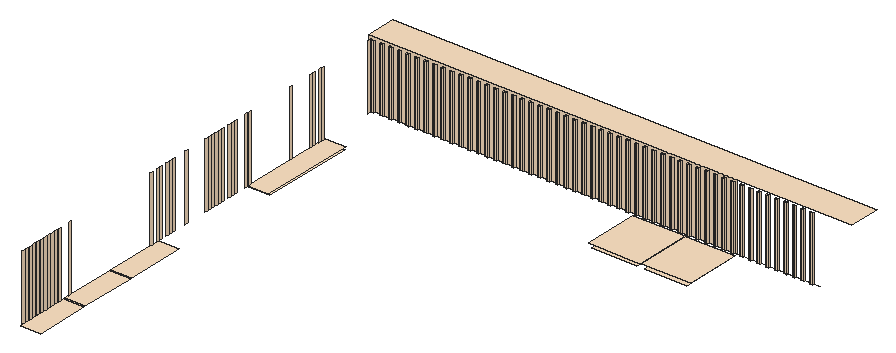
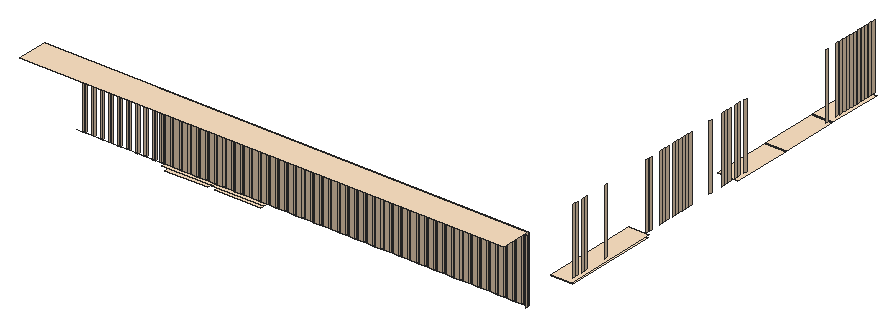
# SketchUp Ruby script. Lengths in inches.
U = 1.inch
M = Sketchup.active_model
def pt(a) = Geom::Point3d.new(a.map { |v| v * U })
def face(e, loops, mat)
  f = e.add_face(loops[0].map { |a| pt(a) })
  loops[1..].each { |l| e.add_face(l.map { |a| pt(a) }).erase! }
  f.material = f.back_material = mat if mat
  f
end
# faces: each face lists its corners as indices into pts; further lists are holes
def faces(e, pts, list, mat = nil) = list.each { |f| face(e, (f[0].is_a?(Array) ? f : [f]).map { |l| l.map { |i| pts[i] } }, mat) }
# xy, xz, yz: faces in a plane at the given z, y or x. An outline is a flat list of corners, or four numbers for a rectangle; further outlines are holes
def ring(l) = l.size == 4 ? [[l[0], l[1]], [l[2], l[1]], [l[2], l[3]], [l[0], l[3]]] : l.each_slice(2).to_a
def flat(e, list, mat, &to3) = list.each { |f| face(e, (f[0].is_a?(Array) ? f : [f]).map { |l| ring(l).map { |u, v| to3.(u, v) } }, mat) }
def xy(e, z, list, mat = nil) = flat(e, list, mat) { |x, y| [x, y, z] }
def xz(e, y, list, mat = nil) = flat(e, list, mat) { |x, z| [x, y, z] }
def yz(e, x, list, mat = nil) = flat(e, list, mat) { |y, z| [x, y, z] }
def lines(e, pts, list) = list.each { |a, b| e.add_line(pt(pts[a]), pt(pts[b])) }
# prism: a flat outline (further loops are holes) pulled along v
def prism(e, loops, v, mat = nil)
  f = face(e, loops, mat); d = Geom::Vector3d.new(v.map { |x| x * U })
  f.pushpull(f.normal.samedirection?(d) ? d.length : -d.length)
end
def box(e, o, s, mat = nil) = prism(e, [[o, [o[0] + s[0], o[1], o[2]], [o[0] + s[0], o[1] + s[1], o[2]], [o[0], o[1] + s[1], o[2]]]], [0, 0, s[2]], mat)
def at(x, y, z, deg = 0) = Geom::Transformation.translation(pt([x, y, z])) * Geom::Transformation.rotation(ORIGIN, Z_AXIS, deg.degrees)
def axes(o, x, y, z) = Geom::Transformation.new([*x, 0, *y, 0, *z, 0, *pt(o).to_a, 1])
def part(name) = M.definitions.add(name)
# library, detail: a bought-in or finely detailed component or shape, given as its bounding box
def library(name, o, s) = part(name).tap { |d| box(d.entities, o, s) }
def detail(e, o, s) = box(e.add_group.entities, o, s)
def put(e, d, t, mat = nil) = e.add_instance(d, t).tap { |i| i.material = mat if mat }
def group(e, t, mat = nil) = e.add_group.tap { |g| g.transformation = t; g.material = mat if mat }.entities
root = M.entities
M.materials.add("[0012_Bisque]").color = [255, 228, 196]
xy(root,98.63,[[103.94,137.53,116.51,154]],"[0012_Bisque]")
xy(root,98.66,[[88.25,137.53,101.61,154]],"[0012_Bisque]")
xy(root,99.09,[[9,109.78,15.0625,137.47]],"[0012_Bisque]")
xy(root,99.5625,[[87.35,137.53,102.51,154],[102.51,137.53,103.01,154],[103.01,137.53,117.4375,154]],"[0012_Bisque]")
xy(root,99.625,[[9,25.15,15.0625,41.09],[9,41.09,15.0625,41.59],[9,41.59,15.0625,58.28],[9,58.78,15.0625,76.4],[9,109.25,15.0625,138]],"[0012_Bisque]")
xy(root,100.32,[[10.09,153.56,10.9,154],[12.6875,153.56,13.5,154],[15.29,153.56,16.1,154],[17.89,153.56,18.7,154],[20.48,153.56,21.3,154],
  [23.08,153.56,23.89,154],[25.68,153.56,26.49,154],[28.28,153.56,29.09,154],[30.88,153.56,31.69,154],[33.48,153.56,34.29,154],
  [36.07,153.56,36.89,154],[38.67,153.56,39.49,154],[41.27,153.56,42.08,154],[43.87,153.56,44.68,154],[46.47,153.56,47.28,154],
  [49.07,153.56,49.88,154],[51.67,153.56,52.48,154],[54.26,153.56,55.08,154],[56.86,153.56,57.68,154],[59.46,153.56,60.27,154],
  [62.06,153.56,62.87,154],[64.66,153.56,65.47,154],[67.26,153.56,68.07,154],[69.85,153.56,70.67,154],[72.45,153.56,73.27,154],
  [75.05,153.56,75.86,154],[77.65,153.56,78.46,154],[80.25,153.56,81.0625,154],[82.85,153.56,83.66,154],[85.45,153.56,86.26,154],
  [88.04,153.56,88.86,154],[90.64,153.56,91.46,154],[93.24,153.56,94.05,154],[95.84,153.56,96.65,154],[98.4375,153.56,99.25,154],
  [101.04,153.56,101.85,154],[103.64,153.56,104.45,154],[106.23,153.56,107.05,154],[108.83,153.56,109.64,154],[111.43,153.56,112.24,154],
  [114.03,153.56,114.84,154],[116.63,153.56,117.44,154],[119.23,153.56,120.04,154],[121.82,153.56,122.64,154],[124.42,153.56,125.24,154],
  [127.02,153.56,127.83,154],[129.62,153.56,130.43,154],[132.22,153.56,133.03,154],[134.82,153.56,135.63,154],[137.42,153.56,138.23,154],
  [140.01,153.56,140.83,154]],"[0012_Bisque]")
xy(root,119.27,[[10.09,153.56,10.9,154],[12.6875,153.56,13.5,154],[15.29,153.56,16.1,154],[17.89,153.56,18.7,154],[20.48,153.56,21.3,154],
  [23.08,153.56,23.89,154],[25.68,153.56,26.49,154],[28.28,153.56,29.09,154],[30.88,153.56,31.69,154],[33.48,153.56,34.29,154],
  [36.07,153.56,36.89,154],[38.67,153.56,39.49,154],[41.27,153.56,42.08,154],[43.87,153.56,44.68,154],[46.47,153.56,47.28,154],
  [49.07,153.56,49.88,154],[51.67,153.56,52.48,154],[54.26,153.56,55.08,154],[56.86,153.56,57.68,154],[59.46,153.56,60.27,154],
  [62.06,153.56,62.87,154],[64.66,153.56,65.47,154],[67.26,153.56,68.07,154],[69.85,153.56,70.67,154],[72.45,153.56,73.27,154],
  [75.05,153.56,75.86,154],[77.65,153.56,78.46,154],[80.25,153.56,81.0625,154],[82.85,153.56,83.66,154],[85.45,153.56,86.26,154],
  [88.04,153.56,88.86,154],[90.64,153.56,91.46,154],[93.24,153.56,94.05,154],[95.84,153.56,96.65,154],[98.4375,153.56,99.25,154],
  [101.04,153.56,101.85,154],[103.64,153.56,104.45,154],[106.23,153.56,107.05,154],[108.83,153.56,109.64,154],[111.43,153.56,112.24,154],
  [114.03,153.56,114.84,154],[116.63,153.56,117.44,154],[119.23,153.56,120.04,154],[121.82,153.56,122.64,154],[124.42,153.56,125.24,154],
  [127.02,153.56,127.83,154],[129.62,153.56,130.43,154],[132.22,153.56,133.03,154],[134.82,153.56,135.63,154],[137.42,153.56,138.23,154],
  [140.01,153.56,140.83,154]],"[0012_Bisque]")
xy(root,120,[[152.125,153.99,152.125,162.99,9,162.99,9,154,117.9375,154]],"[0012_Bisque]")
xz(root,153.56,[[10.09,100.32,10.9,119.27],[12.6875,100.32,13.5,119.27],[15.29,100.32,16.1,119.27],[17.89,100.32,18.7,119.27],[20.48,100.32,21.3,119.27],
  [23.08,100.32,23.89,119.27],[25.68,100.32,26.49,119.27],[28.28,100.32,29.09,119.27],[30.88,100.32,31.69,119.27],[33.48,100.32,34.29,119.27],
  [36.07,100.32,36.89,119.27],[38.67,100.32,39.49,119.27],[41.27,100.32,42.08,119.27],[43.87,100.32,44.68,119.27],[46.47,100.32,47.28,119.27],
  [49.07,100.32,49.88,119.27],[51.67,100.32,52.48,119.27],[54.26,100.32,55.08,119.27],[56.86,100.32,57.68,119.27],[59.46,100.32,60.27,119.27],
  [62.06,100.32,62.87,119.27],[64.66,100.32,65.47,119.27],[67.26,100.32,68.07,119.27],[69.85,100.32,70.67,119.27],[72.45,100.32,73.27,119.27],
  [75.05,100.32,75.86,119.27],[77.65,100.32,78.46,119.27],[80.25,100.32,81.0625,119.27],[82.85,100.32,83.66,119.27],[85.45,100.32,86.26,119.27],
  [88.04,100.32,88.86,119.27],[90.64,100.32,91.46,119.27],[93.24,100.32,94.05,119.27],[95.84,100.32,96.65,119.27],[98.4375,100.32,99.25,119.27],
  [101.04,100.32,101.85,119.27],[103.64,100.32,104.45,119.27],[106.23,100.32,107.05,119.27],[108.83,100.32,109.64,119.27],[111.43,100.32,112.24,119.27],
  [114.03,100.32,114.84,119.27],[116.63,100.32,117.44,119.27],[119.23,100.32,120.04,119.27],[121.82,100.32,122.64,119.27],[124.42,100.32,125.24,119.27],
  [127.02,100.32,127.83,119.27],[129.62,100.32,130.43,119.27],[132.22,100.32,133.03,119.27],[134.82,100.32,135.63,119.27],[137.42,100.32,138.23,119.27],
  [140.01,100.32,140.83,119.27]],"[0012_Bisque]")
xz(root,154,[[9,100.32,9.03,100.32,9.03,119.15,9.59,119.15,9.59,100.32,10.09,100.32,10.09,119.27,10.9,119.27,10.9,100.32,12.6875,100.32,12.6875,119.27,13.5,119.27,13.5,100.32,15.29,100.32,15.29,119.27,16.1,119.27,16.1,100.32,17.89,100.32,17.89,119.27,18.7,119.27,18.7,100.32,20.48,100.32,20.48,119.27,21.3,119.27,21.3,100.32,23.08,100.32,23.08,119.27,23.89,119.27,23.89,100.32,25.68,100.32,25.68,119.27,26.49,119.27,26.49,100.32,28.28,100.32,28.28,119.27,29.09,119.27,29.09,100.32,30.88,100.32,30.88,119.27,31.69,119.27,31.69,100.32,33.48,100.32,33.48,119.27,34.29,119.27,34.29,100.32,36.07,100.32,36.07,119.27,36.89,119.27,36.89,100.32,38.67,100.32,38.67,119.27,39.49,119.27,39.49,100.32,41.27,100.32,41.27,119.27,42.08,119.27,42.08,100.32,43.87,100.32,43.87,119.27,44.68,119.27,44.68,100.32,46.47,100.32,46.47,119.27,47.28,119.27,47.28,100.32,49.07,100.32,49.07,119.27,49.88,119.27,49.88,100.32,51.67,100.32,51.67,119.27,52.48,119.27,52.48,100.32,54.26,100.32,54.26,119.27,55.08,119.27,55.08,100.32,56.86,100.32,56.86,119.27,57.68,119.27,57.68,100.32,59.46,100.32,59.46,119.27,60.27,119.27,60.27,100.32,62.06,100.32,62.06,119.27,62.87,119.27,62.87,100.32,64.66,100.32,64.66,119.27,65.47,119.27,65.47,100.32,67.26,100.32,67.26,119.27,68.07,119.27,68.07,100.32,69.85,100.32,69.85,119.27,70.67,119.27,70.67,100.32,72.45,100.32,72.45,119.27,73.27,119.27,73.27,100.32,75.05,100.32,75.05,119.27,75.86,119.27,75.86,100.32,77.65,100.32,77.65,119.27,78.46,119.27,78.46,100.32,80.25,100.32,80.25,119.27,81.0625,119.27,81.0625,100.32,82.85,100.32,82.85,119.27,83.66,119.27,83.66,100.32,85.45,100.32,85.45,119.27,86.26,119.27,86.26,100.32,88.04,100.32,88.04,119.27,88.86,119.27,88.86,100.32,90.64,100.32,90.64,119.27,91.46,119.27,91.46,100.32,93.24,100.32,93.24,119.27,94.05,119.27,94.05,100.32,95.84,100.32,95.84,119.27,96.65,119.27,96.65,100.32,98.4375,100.32,98.4375,119.27,99.25,119.27,99.25,100.32,101.04,100.32,101.04,119.27,101.85,119.27,101.85,100.32,103.64,100.32,103.64,119.27,104.45,119.27,104.45,100.32,106.23,100.32,106.23,119.27,107.05,119.27,107.05,100.32,108.83,100.32,108.83,119.27,109.64,119.27,109.64,100.32,111.43,100.32,111.43,119.27,112.24,119.27,112.24,100.32,114.03,100.32,114.03,119.27,114.84,119.27,114.84,100.32,116.63,100.32,116.63,119.27,117.44,119.27,117.44,100.32,117.9375,100.32,117.9375,120,9,120]],"[0012_Bisque]")
yz(root,9.5625,[[25.15,100.125,25.98,119.5],[26.4,100.125,27.23,119.5],[27.78,100.125,28.61,119.5],[29.15,100.125,29.98,119.5],[30.53,100.125,31.36,119.5],
  [32.03,100.125,32.86,119.5],[33.28,100.125,34.11,119.5],[34.59,100.125,35.42,119.5],[35.9,100.125,36.73,119.5],[37.21,100.125,38.05,119.5],
  [38.53,100.125,39.36,119.5],[42.46,100.125,43.3,119.5],[72.46,100.125,73.3,119.5],[74.78,100.125,75.61,119.5],[76.03,100.125,76.86,119.5],
  [78.46,100.125,79.3,119.5],[79.65,100.125,80.48,119.5],[80.78,100.125,81.61,119.5],[85.46,100.125,86.3,119.5],[92.9,100.125,93.73,119.5],
  [94.03,100.125,94.86,119.5],[95.21,100.125,96.05,119.5],[96.53,100.125,97.36,119.5],[97.78,100.125,98.61,119.5],[98.96,100.125,99.8,119.5],
  [101.34,100.125,102.17,119.5],[102.53,100.125,103.36,119.5],[103.78,100.125,104.61,119.5],[107.59,100.125,108.42,119.5],[108.96,100.125,109.8,119.5],
  [124.22,100.125,125.05,119.5],[131.54,100.125,132.37,119.5],[132.66,100.125,133.49,119.5],[134.79,100.125,135.62,119.5],[135.85,100.125,136.68,119.5]],"[0012_Bisque]")
yz(root,9.59,[[153.16,99.78,154,119.15]],"[0012_Bisque]")
yz(root,10.09,[[153.56,100.32,154,119.27]],"[0012_Bisque]")
yz(root,10.9,[[153.56,100.32,154,119.27]],"[0012_Bisque]")
yz(root,12.6875,[[153.56,100.32,154,119.27]],"[0012_Bisque]")
yz(root,13.5,[[153.56,100.32,154,119.27]],"[0012_Bisque]")
yz(root,15.29,[[153.56,100.32,154,119.27]],"[0012_Bisque]")
yz(root,16.1,[[153.56,100.32,154,119.27]],"[0012_Bisque]")
yz(root,17.89,[[153.56,100.32,154,119.27]],"[0012_Bisque]")
yz(root,18.7,[[153.56,100.32,154,119.27]],"[0012_Bisque]")
yz(root,20.48,[[153.56,100.32,154,119.27]],"[0012_Bisque]")
yz(root,21.3,[[153.56,100.32,154,119.27]],"[0012_Bisque]")
yz(root,23.08,[[153.56,100.32,154,119.27]],"[0012_Bisque]")
yz(root,23.89,[[153.56,100.32,154,119.27]],"[0012_Bisque]")
yz(root,25.68,[[153.56,100.32,154,119.27]],"[0012_Bisque]")
yz(root,26.49,[[153.56,100.32,154,119.27]],"[0012_Bisque]")
yz(root,28.28,[[153.56,100.32,154,119.27]],"[0012_Bisque]")
yz(root,29.09,[[153.56,100.32,154,119.27]],"[0012_Bisque]")
yz(root,30.88,[[153.56,100.32,154,119.27]],"[0012_Bisque]")
yz(root,31.69,[[153.56,100.32,154,119.27]],"[0012_Bisque]")
yz(root,33.48,[[153.56,100.32,154,119.27]],"[0012_Bisque]")
yz(root,34.29,[[153.56,100.32,154,119.27]],"[0012_Bisque]")
yz(root,36.07,[[153.56,100.32,154,119.27]],"[0012_Bisque]")
yz(root,36.89,[[153.56,100.32,154,119.27]],"[0012_Bisque]")
yz(root,38.67,[[153.56,100.32,154,119.27]],"[0012_Bisque]")
yz(root,39.49,[[153.56,100.32,154,119.27]],"[0012_Bisque]")
yz(root,41.27,[[153.56,100.32,154,119.27]],"[0012_Bisque]")
yz(root,42.08,[[153.56,100.32,154,119.27]],"[0012_Bisque]")
yz(root,43.87,[[153.56,100.32,154,119.27]],"[0012_Bisque]")
yz(root,44.68,[[153.56,100.32,154,119.27]],"[0012_Bisque]")
yz(root,46.47,[[153.56,100.32,154,119.27]],"[0012_Bisque]")
yz(root,47.28,[[153.56,100.32,154,119.27]],"[0012_Bisque]")
yz(root,49.07,[[153.56,100.32,154,119.27]],"[0012_Bisque]")
yz(root,49.88,[[153.56,100.32,154,119.27]],"[0012_Bisque]")
yz(root,51.67,[[153.56,100.32,154,119.27]],"[0012_Bisque]")
yz(root,52.48,[[153.56,100.32,154,119.27]],"[0012_Bisque]")
yz(root,54.26,[[153.56,100.32,154,119.27]],"[0012_Bisque]")
yz(root,55.08,[[153.56,100.32,154,119.27]],"[0012_Bisque]")
yz(root,56.86,[[153.56,100.32,154,119.27]],"[0012_Bisque]")
yz(root,57.68,[[153.56,100.32,154,119.27]],"[0012_Bisque]")
yz(root,59.46,[[153.56,100.32,154,119.27]],"[0012_Bisque]")
yz(root,60.27,[[153.56,100.32,154,119.27]],"[0012_Bisque]")
yz(root,62.06,[[153.56,100.32,154,119.27]],"[0012_Bisque]")
yz(root,62.87,[[153.56,100.32,154,119.27]],"[0012_Bisque]")
yz(root,64.66,[[153.56,100.32,154,119.27]],"[0012_Bisque]")
yz(root,65.47,[[153.56,100.32,154,119.27]],"[0012_Bisque]")
yz(root,67.26,[[153.56,100.32,154,119.27]],"[0012_Bisque]")
yz(root,68.07,[[153.56,100.32,154,119.27]],"[0012_Bisque]")
yz(root,69.85,[[153.56,100.32,154,119.27]],"[0012_Bisque]")
yz(root,70.67,[[153.56,100.32,154,119.27]],"[0012_Bisque]")
yz(root,72.45,[[153.56,100.32,154,119.27]],"[0012_Bisque]")
yz(root,73.27,[[153.56,100.32,154,119.27]],"[0012_Bisque]")
yz(root,75.05,[[153.56,100.32,154,119.27]],"[0012_Bisque]")
yz(root,75.86,[[153.56,100.32,154,119.27]],"[0012_Bisque]")
yz(root,77.65,[[153.56,100.32,154,119.27]],"[0012_Bisque]")
yz(root,78.46,[[153.56,100.32,154,119.27]],"[0012_Bisque]")
yz(root,80.25,[[153.56,100.32,154,119.27]],"[0012_Bisque]")
yz(root,81.0625,[[153.56,100.32,154,119.27]],"[0012_Bisque]")
yz(root,82.85,[[153.56,100.32,154,119.27]],"[0012_Bisque]")
yz(root,83.66,[[153.56,100.32,154,119.27]],"[0012_Bisque]")
yz(root,85.45,[[153.56,100.32,154,119.27]],"[0012_Bisque]")
yz(root,86.26,[[153.56,100.32,154,119.27]],"[0012_Bisque]")
yz(root,88.04,[[153.56,100.32,154,119.27]],"[0012_Bisque]")
yz(root,88.86,[[153.56,100.32,154,119.27]],"[0012_Bisque]")
yz(root,90.64,[[153.56,100.32,154,119.27]],"[0012_Bisque]")
yz(root,91.46,[[153.56,100.32,154,119.27]],"[0012_Bisque]")
yz(root,93.24,[[153.56,100.32,154,119.27]],"[0012_Bisque]")
yz(root,94.05,[[153.56,100.32,154,119.27]],"[0012_Bisque]")
yz(root,95.84,[[153.56,100.32,154,119.27]],"[0012_Bisque]")
yz(root,96.65,[[153.56,100.32,154,119.27]],"[0012_Bisque]")
yz(root,98.4375,[[153.56,100.32,154,119.27]],"[0012_Bisque]")
yz(root,99.25,[[153.56,100.32,154,119.27]],"[0012_Bisque]")
yz(root,101.04,[[153.56,100.32,154,119.27]],"[0012_Bisque]")
yz(root,101.85,[[153.56,100.32,154,119.27]],"[0012_Bisque]")
yz(root,103.64,[[153.56,100.32,154,119.27]],"[0012_Bisque]")
yz(root,104.45,[[153.56,100.32,154,119.27]],"[0012_Bisque]")
yz(root,106.23,[[153.56,100.32,154,119.27]],"[0012_Bisque]")
yz(root,107.05,[[153.56,100.32,154,119.27]],"[0012_Bisque]")
yz(root,108.83,[[153.56,100.32,154,119.27]],"[0012_Bisque]")
yz(root,109.64,[[153.56,100.32,154,119.27]],"[0012_Bisque]")
yz(root,111.43,[[153.56,100.32,154,119.27]],"[0012_Bisque]")
yz(root,112.24,[[153.56,100.32,154,119.27]],"[0012_Bisque]")
yz(root,114.03,[[153.56,100.32,154,119.27]],"[0012_Bisque]")
yz(root,114.84,[[153.56,100.32,154,119.27]],"[0012_Bisque]")
yz(root,116.63,[[153.56,100.32,154,119.27]],"[0012_Bisque]")
yz(root,117.44,[[153.56,100.32,154,119.27]],"[0012_Bisque]")
yz(root,119.23,[[153.56,100.32,154,119.27]],"[0012_Bisque]")
yz(root,120.04,[[153.56,100.32,154,119.27]],"[0012_Bisque]")
yz(root,121.82,[[153.56,100.32,154,119.27]],"[0012_Bisque]")
yz(root,122.64,[[153.56,100.32,154,119.27]],"[0012_Bisque]")
yz(root,124.42,[[153.56,100.32,154,119.27]],"[0012_Bisque]")
yz(root,125.24,[[153.56,100.32,154,119.27]],"[0012_Bisque]")
yz(root,127.02,[[153.56,100.32,154,119.27]],"[0012_Bisque]")
yz(root,127.83,[[153.56,100.32,154,119.27]],"[0012_Bisque]")
yz(root,129.62,[[153.56,100.32,154,119.27]],"[0012_Bisque]")
yz(root,130.43,[[153.56,100.32,154,119.27]],"[0012_Bisque]")
yz(root,132.22,[[153.56,100.32,154,119.27]],"[0012_Bisque]")
yz(root,133.03,[[153.56,100.32,154,119.27]],"[0012_Bisque]")
yz(root,134.82,[[153.56,100.32,154,119.27]],"[0012_Bisque]")
yz(root,135.63,[[153.56,100.32,154,119.27]],"[0012_Bisque]")
yz(root,137.42,[[153.56,100.32,154,119.27]],"[0012_Bisque]")
yz(root,138.23,[[153.56,100.32,154,119.27]],"[0012_Bisque]")
yz(root,140.01,[[153.56,100.32,154,119.27]],"[0012_Bisque]")
yz(root,140.83,[[153.56,100.32,154,119.27]],"[0012_Bisque]")
p = [[117.9375,154,100.32],[119.23,154,100.32],[120.04,154,100.32],[121.82,154,100.32],[122.64,154,100.32],[124.42,154,100.32],
  [125.24,154,100.32],[127.02,154,100.32],[127.83,154,100.32],[129.62,154,100.32],[130.43,154,100.32],[132.22,154,100.32],
  [133.03,154,100.32],[134.82,154,100.32],[135.63,154,100.32],[137.42,154,100.32],[138.23,154,100.32],[140.01,154,100.32],
  [140.83,154,100.32],[142.61,154,100.32]]
lines(root,p,[[0,1],[2,3],[4,5],[6,7],[8,9],[10,11],[12,13],[14,15],[16,17],[18,19]])
